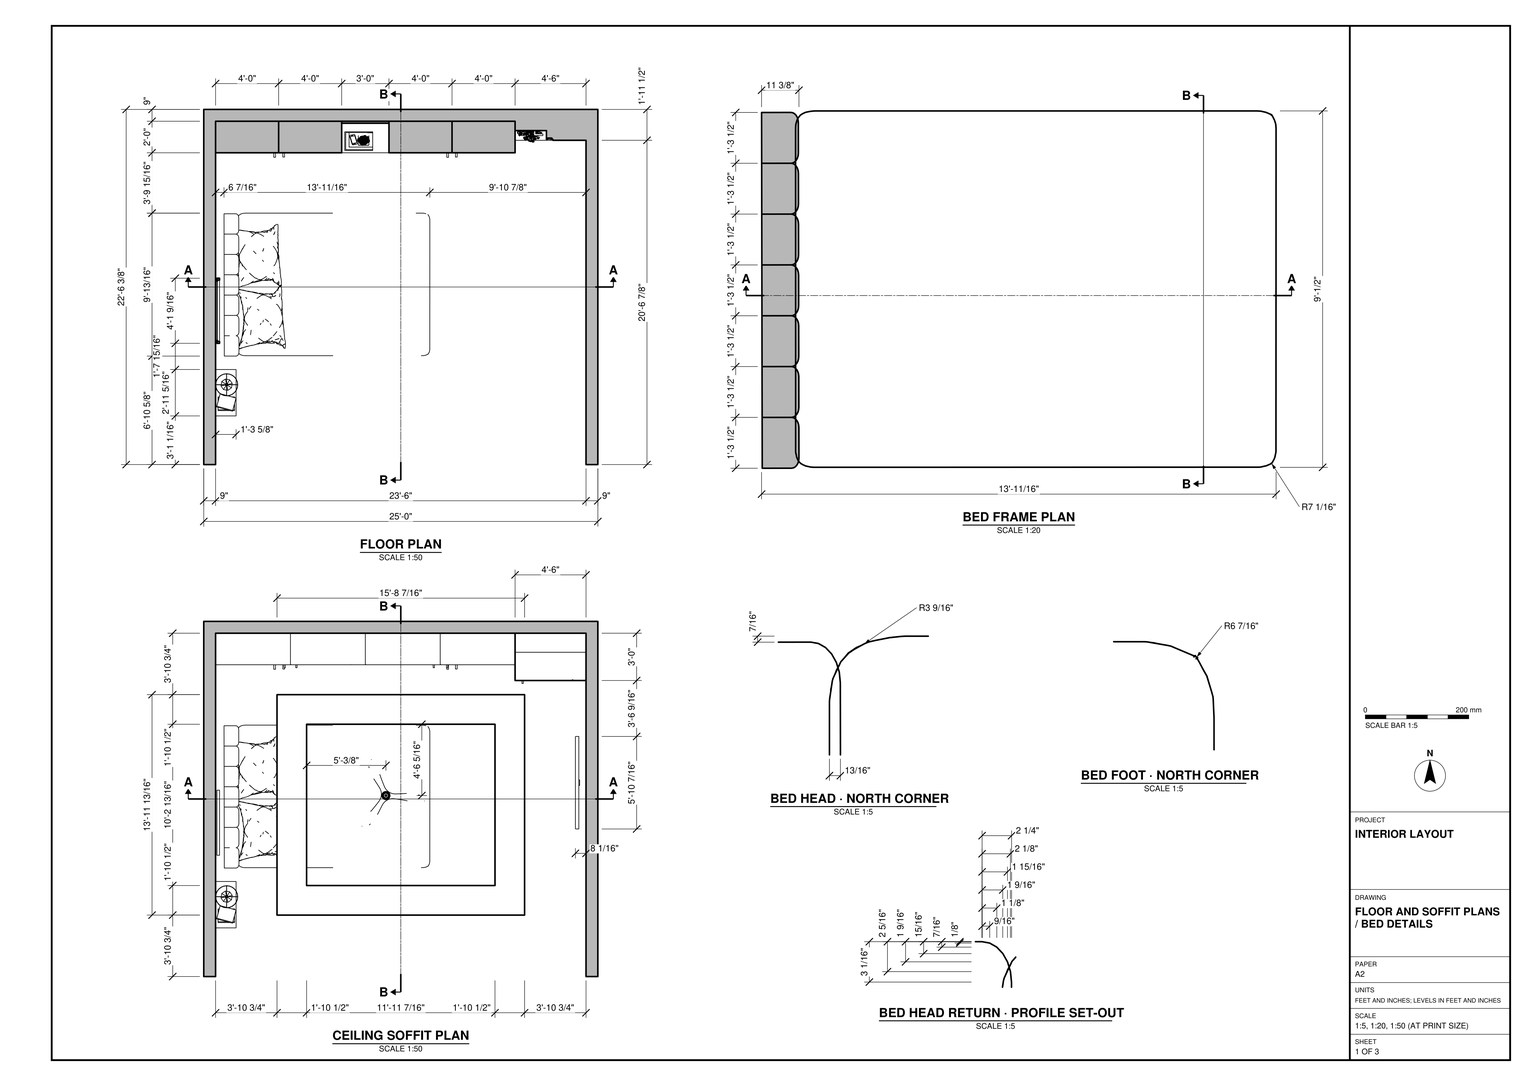
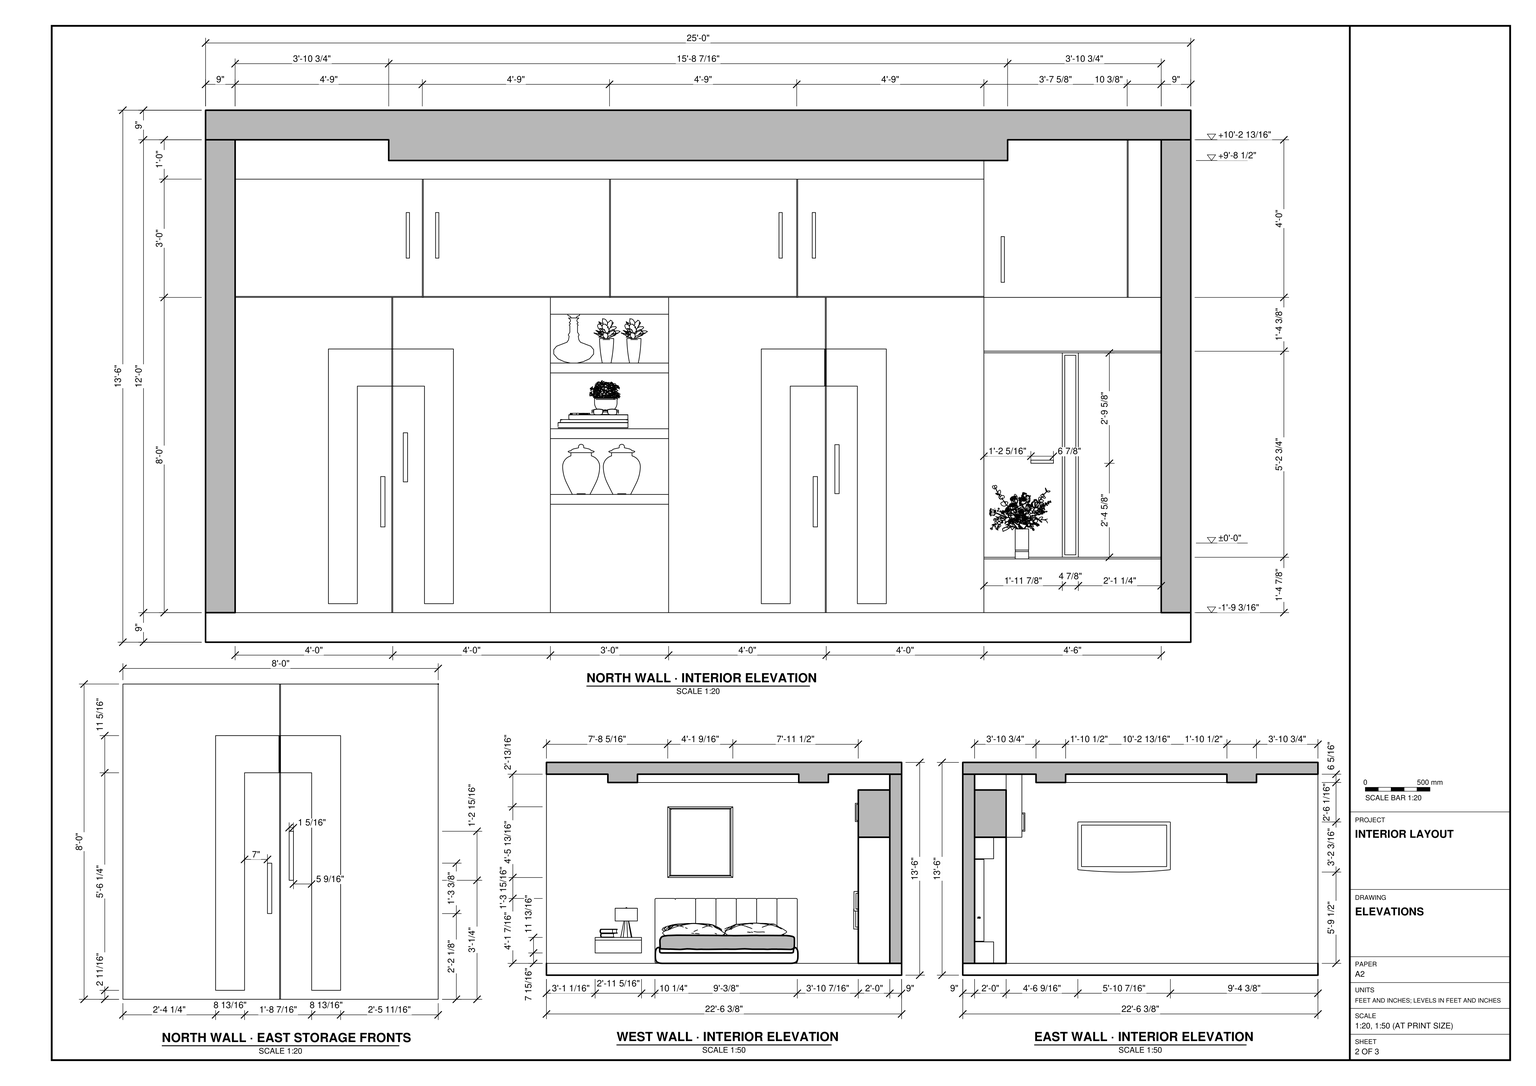
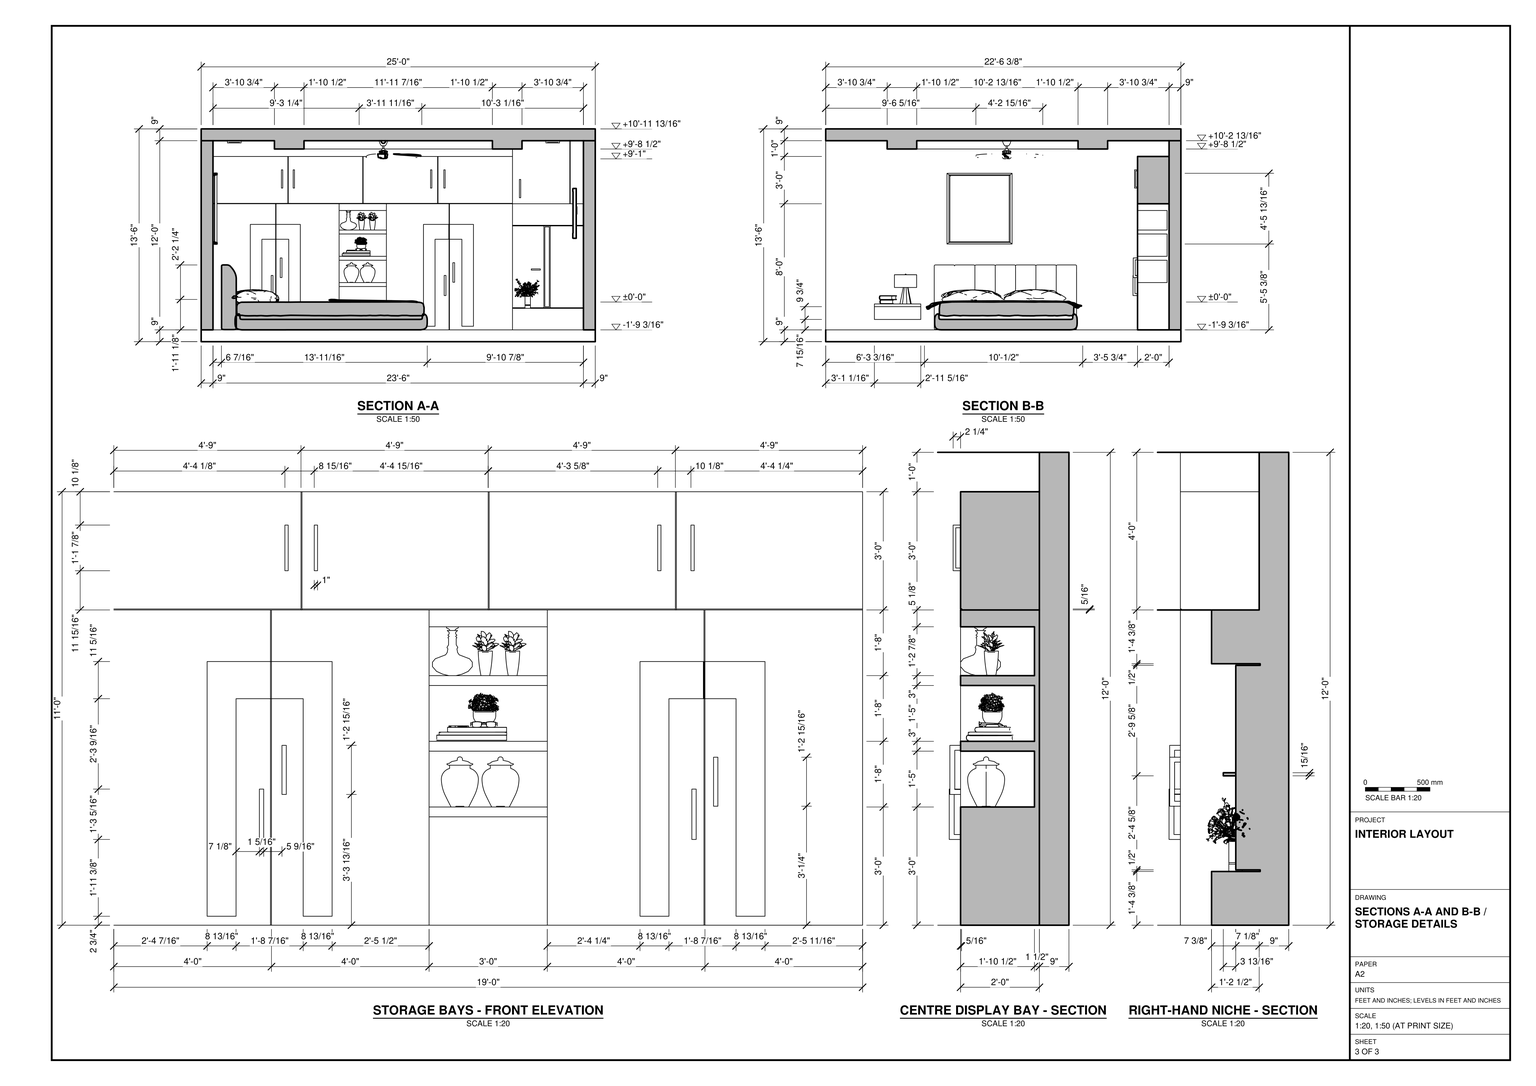
Build the bedroom interior in SketchUp from task_files/diagram_01.pdf. Work in feet and inches. The model is 25'-0" wide from west to east, 22'-6 3/8" deep from north to south and 13'-6" high. Use the single storey datum of ±0'-0" shown in the sections.

Form the floor slab, ceiling slab and 9" walls on the north, east and west sides, leaving the south side open as drawn. Follow the ceiling soffit plan and both sections to form the rectangular dropped band around the recessed centre. Place the ceiling fan within that recess at the position shown.

Run the fitted storage across the north wall. Distinguish the tall paired fronts, central display shelves, upper cupboards and stepped niche at the east end. Use the storage elevations for the front divisions, inset outlines and offset handles, and the bay sections for shelf depths and projections. Set the platform bed with its segmented head toward the west wall and its rounded foot toward the east. Include the mattress, the bedside unit south of the head, the framed panel above the bed and the screen opposite it. Decor and loose items such as lamps, cushions, plants and books may be any suitable library components, for example from 3D Warehouse.

Keep the walls, slabs and soffit, and each furniture or joinery piece, in separate groups or components. Use components for repeated parts. Save one SketchUp model as output_files/bedroom_with_fitted_storage_and_a_platform_bed.skp.

# SketchUp Ruby script. Lengths in inches.
U = 1.inch
M = Sketchup.active_model
def pt(a) = Geom::Point3d.new(a.map { |v| v * U })
def face(e, loops, mat)
  f = e.add_face(loops[0].map { |a| pt(a) })
  loops[1..].each { |l| e.add_face(l.map { |a| pt(a) }).erase! }
  f.material = f.back_material = mat if mat
  f
end
# faces: each face lists its corners as indices into pts; further lists are holes
def faces(e, pts, list, mat = nil) = list.each { |f| face(e, (f[0].is_a?(Array) ? f : [f]).map { |l| l.map { |i| pts[i] } }, mat) }
# xy, xz, yz: faces in a plane at the given z, y or x. An outline is a flat list of corners, or four numbers for a rectangle; further outlines are holes
def ring(l) = l.size == 4 ? [[l[0], l[1]], [l[2], l[1]], [l[2], l[3]], [l[0], l[3]]] : l.each_slice(2).to_a
def flat(e, list, mat, &to3) = list.each { |f| face(e, (f[0].is_a?(Array) ? f : [f]).map { |l| ring(l).map { |u, v| to3.(u, v) } }, mat) }
def xy(e, z, list, mat = nil) = flat(e, list, mat) { |x, y| [x, y, z] }
def xz(e, y, list, mat = nil) = flat(e, list, mat) { |x, z| [x, y, z] }
def yz(e, x, list, mat = nil) = flat(e, list, mat) { |y, z| [x, y, z] }
def lines(e, pts, list) = list.each { |a, b| e.add_line(pt(pts[a]), pt(pts[b])) }
# prism: a flat outline (further loops are holes) pulled along v
def prism(e, loops, v, mat = nil)
  f = face(e, loops, mat); d = Geom::Vector3d.new(v.map { |x| x * U })
  f.pushpull(f.normal.samedirection?(d) ? d.length : -d.length)
end
def box(e, o, s, mat = nil) = prism(e, [[o, [o[0] + s[0], o[1], o[2]], [o[0] + s[0], o[1] + s[1], o[2]], [o[0], o[1] + s[1], o[2]]]], [0, 0, s[2]], mat)
def at(x, y, z, deg = 0) = Geom::Transformation.translation(pt([x, y, z])) * Geom::Transformation.rotation(ORIGIN, Z_AXIS, deg.degrees)
def axes(o, x, y, z) = Geom::Transformation.new([*x, 0, *y, 0, *z, 0, *pt(o).to_a, 1])
def part(name) = M.definitions.add(name)
# library, detail: a bought-in or finely detailed component or shape, given as its bounding box
def library(name, o, s) = part(name).tap { |d| box(d.entities, o, s) }
def detail(e, o, s) = box(e.add_group.entities, o, s)
def put(e, d, t, mat = nil) = e.add_instance(d, t).tap { |i| i.material = mat if mat }
def group(e, t, mat = nil) = e.add_group.tap { |g| g.transformation = t; g.material = mat if mat }.entities
root = M.entities
M.materials.add("Ceramic White").color = [255, 255, 255]
M.materials.add("Generic\#1").color = [232, 226, 159]
M.materials.add("[Color M07]").color = [58, 58, 58]
M.materials.add("[Tile Limestone Large]").color = [236, 249, 228]
M.materials.add("[Wood Bamboo]").color = [153, 90, 37]
c1 = library("Flower+Arrangement",[-12.45,-7.69,-0.03],[24.36,19.47,24.52])
c2 = library("00000871-book1",[-1.17,-10.85,-0.02],[14.86,13.34,6.32])
c3 = library("Lidded jar",[0,0,0],[13.42,13.42,18.18])
c4 = library("books",[6.19,-1.3125,-0.22],[15.35,11.9,12.07])
c5 = library("Lamp+10 (1)",[0,0,0],[16.92,16.92,22.79])
c6 = library("Untitled",[82.71,28.87,-11.8125],[39.77,1.97,25.2])
c7 = library("sri rejeki",[-5.27,-3.99,-0.125],[72.84,72.27,70.8])
c8 = library("Tlon Light 450 Ceiling 152 006",[-8.86,-8.86,-3.78],[17.72,17.72,3.56])
c9 = library("Avation+Styled+Ceiling+Fan_JSB",[-19.77,-29.63,-13.8125],[51.59,58.16,13.8125])
c10 = library("Group\#9",[0,0,0],[159.9,159.9,209.38])
c11 = library("Group\#50",[-3.59,0,-0.01],[91.02,69.39,39.65])
c12 = library("Group\#4",[0,0,0],[11.81,11.74,23.62])
c13 = library("Group\#16",[-1.58,-1.2,0],[21.85,21.68,32.68])
c14 = part("Agrupar\#12")
xy(c14.entities,0,[[0,13.9375,0,31.5,0.51,30.98,0.51,14.45]])
xy(c14.entities,1.0625,[[0.51,14.45,0.51,30.98,0.79,30.71,0.79,14.72]])
xy(c14.entities,1.26,[[0,13.9375,0.79,14.72,0.79,30.71,0,31.5]])
yz(c14.entities,0,[[13.9375,0,31.5,1.26]])
yz(c14.entities,0.51,[[14.45,0,30.98,1.0625]])
yz(c14.entities,0.79,[[14.72,1.0625,30.71,1.26]])
p = [[0.79,14.72,1.26],[0,13.9375,1.26],[0,13.9375,0],[0.51,14.45,0],[0.51,14.45,1.0625],[0.79,14.72,1.0625],
  [0,31.5,1.26],[0.79,30.71,1.26],[0.79,30.71,1.0625],[0.51,30.98,1.0625],[0.51,30.98,0],[0,31.5,0]]
faces(c14.entities,p,[[0,1,2,3,4,5],[6,7,8,9,10,11]])
c15 = part("Agrupar\#31")
xy(c15.entities,0,[[0,6.85,0,31.5,0.51,30.98,0.51,7.36]])
xy(c15.entities,1.0625,[[0.51,7.36,0.51,30.98,0.79,30.71,0.79,7.64]])
xy(c15.entities,1.26,[[0,6.85,0.79,7.64,0.79,30.71,0,31.5]])
yz(c15.entities,0,[[6.85,0,31.5,1.26]])
yz(c15.entities,0.51,[[7.36,0,30.98,1.0625]])
yz(c15.entities,0.79,[[7.64,1.0625,30.71,1.26]])
p = [[0.79,7.64,1.26],[0,6.85,1.26],[0,6.85,0],[0.51,7.36,0],[0.51,7.36,1.0625],[0.79,7.64,1.0625],
  [0,31.5,1.26],[0.79,30.71,1.26],[0.79,30.71,1.0625],[0.51,30.98,1.0625],[0.51,30.98,0],[0,31.5,0]]
faces(c15.entities,p,[[0,1,2,3,4,5],[6,7,8,9,10,11]])
c16 = part("Agrupar\#29")
put(c16.entities,c14,at(0,-13.9375,0))
put(c16.entities,c15,at(31.5,0,0,90))
put(c16.entities,c14,at(24.65,31.5,0,-180))
put(c16.entities,c15,at(-6.85,17.56,0,-90))
xy(root,-9,[[0,0,300,270.375]],"[Tile Limestone Large]")
xy(root,0,[[0,0,9,0,9,261.375,237,261.375,237,246.875,291,246.875,291,0,300,0,300,270.375,0,270.375],[9,237.375,56.7,237.375,56.7,237.68,57,237.68,57,261.375,9,261.375],[57,237.375,105,261.375],[105,237.375,141,261.375],[141,237.375,188.7,237.375,188.7,237.68,189,237.68,189,261.375,141,261.375],
  [189,237.375,237,261.375]])
xy(root,7.92,[[9,37.05,24.62,72.37]])
xy(root,16.36,[[260.875,246.875,263.875,261.67],[263.875,246.875,291,261.67]])
xy(root,16.36,[[237,246.875,260.875,261.67]],"[Wood Bamboo]")
xy(root,16.86,[[265.75,246.875,265.75,251.4375,263.875,261.67,291,261.67,291,246.875],[260.875,247.625,260.875,261.67,263.875,261.67,265.75,251.4375,265.75,247.625],[237,254.25,260.875,261.67]])
xy(root,17.61,[[261.625,247.625,265,248.5625]])
xy(root,17.67,[[9,37.05,24.62,72.37]])
xy(root,19.73,[[9,37.05,24.62,72.37]])
xy(root,26.11,[[53.32,233.93,54.64,237.375],[185.01,233.93,186.32,237.375]],"[Color M07]")
xy(root,27.61,[[53.32,235.43,54.64,237.375],[185.01,235.43,186.32,237.375]],"[Color M07]")
xy(root,36,[[105,237.375,141,259.875]],"[Wood Bamboo]")
xy(root,36.23,[[191.62,234.13,192.93,237.375]],"[Color M07]")
xy(root,37.73,[[191.62,235.63,192.93,237.375]],"[Color M07]")
xy(root,39.82,[[60.21,234.12,61.52,237.375]],"[Color M07]")
xy(root,39.95,[[53.32,235.43,54.64,237.375],[185.01,235.43,186.32,237.375]],"[Color M07]")
xy(root,41.32,[[60.21,235.62,61.52,237.375]],"[Color M07]")
xy(root,41.45,[[53.32,233.93,54.64,237.375],[185.01,233.93,186.32,237.375]],"[Color M07]")
xy(root,45.49,[[251.3125,250.45,251.3125,254.25,252.625,254.25,252.625,251.76,258.18,251.76,258.18,250.45]],"[Color M07]")
xy(root,46.44,[[251.3125,250.45,258.18,250.45,258.18,251.76,252.625,251.76,252.625,254.25,251.3125,254.25]],"[Color M07]")
xy(root,49.66,[[191.62,235.63,192.93,237.375]],"[Color M07]")
xy(root,51.16,[[191.62,234.13,192.93,237.375]],"[Color M07]")
xy(root,53,[[105,237.375,141,259.875]])
xy(root,53.27,[[60.21,235.62,61.52,237.375]])
xy(root,54.77,[[60.21,234.12,61.52,237.375]],"[Color M07]")
xy(root,56,[[105,237.375,141,259.875]],"[Wood Bamboo]")
xy(root,73,[[105,237.375,141,259.875]])
xy(root,76,[[105,237.375,141,259.875]],"[Wood Bamboo]")
xy(root,78.375,[[261.625,247.625,265,248.5625]])
xy(root,79.125,[[265.75,246.875,291,246.875,291,261.67,263.875,261.67,265.75,251.4375],[260.875,247.625,265.75,247.625,265.75,251.4375,263.875,261.67,260.875,261.67],[237,254.25,260.875,261.67]])
xy(root,79.625,[[237,246.875,260.875,261.67],[260.875,246.875,263.875,261.67],[263.875,246.875,291,261.67]],"[Wood Bamboo]")
xy(root,90.875,[[105,237.375,141,259.875]])
xy(root,96,[[9,237.375,56.7,237.68],[57,237.375,66,237.68],[66,237.375,66.3,237.68],[66.3,237.375,105,237.68],[105,237.375,123,237.68],
  [123,237.375,123.3,237.68],[123.3,237.375,141,237.68],[141,237.375,180,237.68],[180,237.375,180.3,237.68],[180.3,237.375,188.7,237.68],
  [189,237.375,237,237.68],[9,237.68,57,261.375],[57,237.68,66,261.375],[66,237.68,105,261.375],[105,237.68,123,261.375],
  [123,237.68,141,261.375],[141,237.68,180,261.375],[180,237.68,189,261.375],[189,237.68,237,261.375],[237,246.875,291,261.375]])
xy(root,96,[[237,225.375,237,246.875,291,246.875,291,225.375,280.9375,225.375,280.9375,225.68,280.64,225.68,280.64,225.375]],"[Wood Bamboo]")
xy(root,96.3,[[9,237.375,57,237.68],[57,237.375,66,237.68],[66.3,237.375,105,237.68],[105,237.375,123,237.68],[123.3,237.375,141,237.68],
  [141,237.375,180,237.68],[180.3,237.375,189,237.68],[189,237.375,237,237.68]])
xy(root,100.58,[[242.25,223.09,243.25,225.375]],"[Color M07]")
xy(root,101.4,[[242.25,223.9,243.25,225.375]],"[Color M07]")
xy(root,107.95,[[61.1,235.11,62.1,237.375],[70.03,235.11,71.03,237.375],[174.61,235.11,175.61,237.375],[184.73,235.11,185.73,237.375]],"[Color M07]")
xy(root,108.76,[[61.1,235.92,62.1,237.375],[70.03,235.92,71.03,237.375],[174.61,235.92,175.61,237.375],[184.73,235.92,185.73,237.375]],"[Color M07]")
xy(root,113.71,[[242.25,223.9,243.25,225.375]])
xy(root,114.52,[[242.25,223.09,243.25,225.375]],"[Color M07]")
xy(root,121.04,[[61.1,235.92,62.1,237.375],[70.03,235.92,71.03,237.375]])
xy(root,121.04,[[174.61,235.92,175.61,237.375],[184.73,235.92,185.73,237.375]],"[Color M07]")
xy(root,121.85,[[184.73,235.11,185.73,237.375]])
xy(root,121.85,[[61.1,235.11,62.1,237.375],[70.03,235.11,71.03,237.375],[174.61,235.11,175.61,237.375]],"[Color M07]")
xy(root,132,[[9,237.375,66,261.375],[66.3,237.375,123,237.375,123,261.375,66,261.375,66,237.68,66.3,237.68],[123.3,237.375,180,237.375,180,261.375,123,261.375,123,237.68,123.3,237.68],[180.3,237.375,237,237.375,237,261.375,180,261.375,180,237.68,180.3,237.68]],"[Wood Bamboo]")
xy(root,137.6875,[[[55.77,46.77,244.23,214.61],[78.29,69.29,221.71,192.08]]],"Generic\#1")
xy(root,144,[[0,0,0,270.375,300,270.375,300,0,291,0,291,261.375,9,261.375,9,0],[237,225.375,237,261.375,291,261.375,291,225.375,280.9375,225.375,280.9375,225.68,280.64,225.68,280.64,225.375]])
xy(root,144,[[[9,0,9,261.375,237,261.375,237,225.375,280.64,225.375,280.64,225.68,280.9375,225.68,280.9375,225.375,291,225.375,291,0],[55.77,46.77,244.23,214.61]],[78.29,69.29,221.71,192.08]],"Generic\#1")
xy(root,153,[[0,0,300,270.375]])
xz(root,0,[[0,-9,300,0],[0,0,9,144],[291,0,300,144],[0,144,300,153]])
xz(root,37.05,[[9,7.92,24.62,17.67],[9,17.67,24.62,19.73]])
xz(root,46.77,[[55.77,137.6875,244.23,144]],"Generic\#1")
xz(root,69.29,[[78.29,137.6875,221.71,144]])
xz(root,72.37,[[9,7.92,24.62,17.67],[9,17.67,24.62,19.73]])
xz(root,192.08,[[78.29,137.6875,221.71,144]],"Generic\#1")
xz(root,214.61,[[55.77,137.6875,190.23,144],[190.23,137.6875,234.17,144],[234.17,137.6875,244.23,144]])
xz(root,223.09,[[242.25,100.58,243.25,114.52]],"[Color M07]")
xz(root,223.9,[[242.25,101.4,243.25,113.71]])
xz(root,225.375,[[242.25,113.71,243.25,114.52]])
xz(root,225.375,[[[237,96,280.64,144],[242.25,113.71,243.25,114.52],[242.25,100.58,243.25,101.4]],[280.9375,96,291,144]],"[Wood Bamboo]")
xz(root,225.68,[[280.64,96,280.9375,144]])
xz(root,233.93,[[53.32,26.11,54.64,41.45],[185.01,26.11,186.32,41.45]],"[Color M07]")
xz(root,234.12,[[60.21,39.82,61.52,54.77]],"[Color M07]")
xz(root,234.13,[[191.62,36.23,192.93,51.16]],"[Color M07]")
xz(root,235.11,[[61.1,107.95,62.1,121.85],[70.03,107.95,71.03,121.85],[174.61,107.95,175.61,121.85],[184.73,107.95,185.73,121.85]],"[Color M07]")
xz(root,235.43,[[53.32,27.61,54.64,39.95],[185.01,27.61,186.32,39.95]])
xz(root,235.62,[[60.21,41.32,61.52,53.27]])
xz(root,235.63,[[191.62,37.73,192.93,49.66]])
xz(root,235.92,[[61.1,108.76,62.1,121.04],[70.03,108.76,71.03,121.04],[174.61,108.76,175.61,121.04],[184.73,108.76,185.73,121.04]])
xz(root,237.375,[[37.41,2.73,46.22,2.73,46.22,68.98,56.7,68.98,56.7,80.29,37.41,80.29],[66.66,2.73,75.47,2.73,75.47,80.29,57,80.29,57,68.98,66.66,68.98],[169.22,2.73,178.04,2.73,178.04,68.98,188.51,68.98,188.51,80.29,169.22,80.29],[198.47,2.73,207.29,2.73,207.29,80.29,189,80.29,189,68.98,198.47,68.98],[53.32,39.95,54.64,41.45],
  [185.01,39.95,186.32,41.45],[191.62,49.66,192.93,51.16],[60.21,53.27,61.52,54.77],[56.7,68.98,57,80.29],[188.8125,68.98,189,80.29],
  [61.1,121.04,62.1,121.85],[70.03,121.04,71.03,121.85],[174.61,121.04,175.61,121.85],[184.73,121.04,185.73,121.85]])
xz(root,237.375,[[[9,0,56.7,0,56.7,68.98,46.22,68.98,46.22,2.73,37.41,2.73,37.41,80.29,56.7,80.29,56.7,96,9,96],[53.32,39.95,54.64,41.45],[53.32,26.11,54.64,27.61]],[[57,0,105,0,105,96,57,96,57,80.29,75.47,80.29,75.47,2.73,66.66,2.73,66.66,68.98,57,68.98],[60.21,53.27,61.52,54.77],[60.21,39.82,61.52,41.32]],[105,0,141,33],[[141,0,188.7,96],[169.22,2.73,169.22,80.29,188.51,80.29,188.51,68.98,178.04,68.98,178.04,2.73],[185.01,39.95,186.32,41.45],[185.01,26.11,186.32,27.61]],[[189,0,237,0,237,96,189,96,189,80.29,207.29,80.29,207.29,2.73,198.47,2.73,198.47,68.98,189,68.98],[191.62,49.66,192.93,51.16],[191.62,36.23,192.93,37.73]],
  [105,33,141,36],[105,53,141,56],[105,73,141,76],[105,90.875,141,96],[[9,96.3,66,132],[61.1,121.04,62.1,121.85],[61.1,107.95,62.1,108.76]],
  [[66.3,96.3,123,132],[70.03,121.04,71.03,121.85],[70.03,107.95,71.03,108.76]],[[123.3,96.3,180,132],[174.61,121.04,175.61,121.85],[174.61,107.95,175.61,108.76]],[[180.3,96.3,237,132],[184.73,121.04,185.73,121.85],[184.73,107.95,185.73,108.76]]],"[Wood Bamboo]")
xz(root,237.68,[[56.7,0,57,96],[188.7,0,189,96],[9,96,66,96.3],[66,96,66.3,132],[66.3,96,123,96.3],
  [123,96,123.3,132],[123.3,96,180,96.3],[180,96,180.3,132],[180.3,96,237,96.3]])
xz(root,246.875,[[237,0,291,16.36],[265.75,16.86,291,79.125],[237,79.625,291,96]],"[Wood Bamboo]")
xz(root,247.625,[[[260.875,16.86,265.75,79.125],[261.625,17.61,265,78.375]]],"[Wood Bamboo]")
xz(root,248.5625,[[261.625,17.61,265,78.375]],"[Wood Bamboo]")
xz(root,250.45,[[251.3125,45.49,258.18,46.44]],"[Color M07]")
xz(root,251.76,[[252.625,45.49,258.18,46.44]])
xz(root,254.25,[[251.3125,45.49,252.625,46.44]])
xz(root,254.25,[[[237,16.86,260.875,79.125],[251.3125,45.49,252.625,46.44]]],"[Wood Bamboo]")
xz(root,259.875,[[105,36,141,53],[105,56,141,73],[105,76,141,90.875]],"[Wood Bamboo]")
xz(root,261.375,[[9,0,57,96],[57,0,105,96],[105,0,141,96],[141,0,189,96],[189,0,237,96],
  [9,96,66,132],[66,96,123,132],[123,96,180,132],[180,96,237,132],[237,96,291,144]])
xz(root,261.375,[[9,132,237,144]],"[Wood Bamboo]")
xz(root,261.67,[[237,16.36,291,16.86],[237,79.125,291,79.625]])
xz(root,270.375,[[0,0,300,144],[0,144,300,153]])
xz(root,270.375,[[0,-9,300,0]],"Generic\#1")
yz(root,0,[[0,-9,270.375,0],[0,0,270.375,144],[0,144,270.375,153]])
yz(root,9,[[237.375,0,261.375,96],[37.05,7.92,72.37,17.67],[37.05,17.67,72.37,19.73],[237.68,96,261.375,96,261.375,132,237.375,132,237.375,96.3,237.68,96.3]])
yz(root,9,[[[0,0,237.375,0,237.375,96,237.68,96,237.68,96.3,237.375,96.3,237.375,132,261.375,132,261.375,144,0,144],[37.05,7.92,72.37,19.73]]],"Generic\#1")
yz(root,24.62,[[37.05,7.92,72.37,17.67],[37.05,17.67,72.37,19.73]])
yz(root,53.32,[[233.93,26.11,233.93,41.45,237.375,41.45,237.375,39.95,235.43,39.95,235.43,27.61,237.375,27.61,237.375,26.11]],"[Color M07]")
yz(root,54.64,[[233.93,26.11,237.375,26.11,237.375,27.61,235.43,27.61,235.43,39.95,237.375,39.95,237.375,41.45,233.93,41.45]],"[Color M07]")
yz(root,55.77,[[46.77,137.6875,214.61,144]])
yz(root,56.7,[[237.375,0,237.68,96]])
yz(root,57,[[237.375,0,237.68,96],[237.68,0,261.375,96]])
yz(root,60.21,[[234.12,39.82,234.12,54.77,237.375,54.77,237.375,53.27,235.62,53.27,235.62,41.32,237.375,41.32,237.375,39.82]],"[Color M07]")
yz(root,61.1,[[235.11,107.95,235.11,121.85,237.375,121.85,237.375,121.04,235.92,121.04,235.92,108.76,237.375,108.76,237.375,107.95]],"[Color M07]")
yz(root,61.52,[[234.12,39.82,237.375,39.82,237.375,41.32,235.62,41.32,235.62,53.27,237.375,53.27,237.375,54.77,234.12,54.77]],"[Color M07]")
yz(root,62.1,[[235.11,107.95,237.375,107.95,237.375,108.76,235.92,108.76,235.92,121.04,237.375,121.04,237.375,121.85,235.11,121.85]],"[Color M07]")
yz(root,66,[[237.68,96,261.375,132],[237.375,96.3,237.68,132]])
yz(root,66.3,[[237.375,96.3,237.68,132]])
yz(root,70.03,[[235.11,107.95,235.11,121.85,237.375,121.85,237.375,121.04,235.92,121.04,235.92,108.76,237.375,108.76,237.375,107.95]],"[Color M07]")
yz(root,71.03,[[235.11,107.95,237.375,107.95,237.375,108.76,235.92,108.76,235.92,121.04,237.375,121.04,237.375,121.85,235.11,121.85]],"[Color M07]")
yz(root,78.29,[[69.29,137.6875,192.08,144]],"Generic\#1")
yz(root,105,[[237.375,0,261.375,0,261.375,96,237.375,96,237.375,90.875,259.875,90.875,259.875,76,237.375,76,237.375,73,259.875,73,259.875,56,237.375,56,237.375,53,259.875,53,259.875,36,237.375,36]])
yz(root,105,[[237.375,36,259.875,53],[237.375,56,259.875,73],[237.375,76,259.875,90.875]],"[Wood Bamboo]")
yz(root,123,[[237.68,96,261.375,132],[237.375,96.3,237.68,132]])
yz(root,123.3,[[237.375,96.3,237.68,132]])
yz(root,141,[[237.375,0,261.375,0,261.375,96,237.375,96,237.375,90.875,259.875,90.875,259.875,76,237.375,76,237.375,73,259.875,73,259.875,56,237.375,56,237.375,53,259.875,53,259.875,36,237.375,36]])
yz(root,141,[[237.375,36,259.875,53],[237.375,56,259.875,73],[237.375,76,259.875,90.875]],"[Wood Bamboo]")
yz(root,174.61,[[235.11,107.95,235.11,121.85,237.375,121.85,237.375,121.04,235.92,121.04,235.92,108.76,237.375,108.76,237.375,107.95]],"[Color M07]")
yz(root,175.61,[[235.11,107.95,237.375,107.95,237.375,108.76,235.92,108.76,235.92,121.04,237.375,121.04,237.375,121.85,235.11,121.85]],"[Color M07]")
yz(root,180,[[237.68,96,261.375,132],[237.375,96.3,237.68,132]])
yz(root,180.3,[[237.375,96.3,237.68,132]])
yz(root,184.73,[[235.11,107.95,235.11,121.85,237.375,121.85,237.375,121.04,235.92,121.04,235.92,108.76,237.375,108.76,237.375,107.95]],"[Color M07]")
yz(root,185.01,[[233.93,26.11,233.93,41.45,237.375,41.45,237.375,39.95,235.43,39.95,235.43,27.61,237.375,27.61,237.375,26.11]],"[Color M07]")
yz(root,185.73,[[235.11,107.95,237.375,107.95,237.375,108.76,235.92,108.76,235.92,121.04,237.375,121.04,237.375,121.85,235.11,121.85]],"[Color M07]")
yz(root,186.32,[[233.93,26.11,237.375,26.11,237.375,27.61,235.43,27.61,235.43,39.95,237.375,39.95,237.375,41.45,233.93,41.45]],"[Color M07]")
yz(root,188.7,[[237.375,0,237.68,96]])
yz(root,189,[[237.375,0,237.68,96],[237.68,0,261.375,96]])
yz(root,191.62,[[234.13,36.23,234.13,51.16,237.375,51.16,237.375,49.66,235.63,49.66,235.63,37.73,237.375,37.73,237.375,36.23]],"[Color M07]")
yz(root,192.93,[[234.13,36.23,237.375,36.23,237.375,37.73,235.63,37.73,235.63,49.66,237.375,49.66,237.375,51.16,234.13,51.16]],"[Color M07]")
yz(root,221.71,[[69.29,137.6875,192.08,144]],"Generic\#1")
yz(root,237,[[246.875,0,261.375,16.36],[261.375,16.36,261.67,16.86],[254.25,16.86,261.375,79.125],[261.375,79.125,261.67,79.625],[246.875,79.625,261.375,96],
  [237.68,96,237.68,96.3,237.375,96.3,237.375,132,261.375,132,261.375,96]])
yz(root,237,[[237.375,0,246.875,0,246.875,16.36,261.375,16.36,261.375,16.86,254.25,16.86,254.25,79.125,261.375,79.125,261.375,79.625,246.875,79.625,246.875,96,237.375,96],[225.375,96,225.375,144,237.375,144,237.375,96.3,237.68,96.3,237.68,96],[237.375,132,261.375,144]],"[Wood Bamboo]")
yz(root,242.25,[[223.09,100.58,223.09,114.52,225.375,114.52,225.375,113.71,223.9,113.71,223.9,101.4,225.375,101.4,225.375,100.58]],"[Color M07]")
yz(root,243.25,[[223.09,100.58,225.375,100.58,225.375,101.4,223.9,101.4,223.9,113.71,225.375,113.71,225.375,114.52,223.09,114.52]],"[Color M07]")
yz(root,244.23,[[46.77,137.6875,214.61,144]])
yz(root,251.3125,[[250.45,45.49,254.25,46.44]],"[Color M07]")
yz(root,252.625,[[251.76,45.49,254.25,46.44]],"[Color M07]")
yz(root,258.18,[[250.45,45.49,251.76,46.44]])
yz(root,260.875,[[247.625,16.86,254.25,79.125]],"[Wood Bamboo]")
yz(root,261.625,[[247.625,17.61,248.5625,78.375]])
yz(root,265,[[247.625,17.61,248.5625,78.375]])
yz(root,265.75,[[246.875,16.86,247.625,79.125]])
yz(root,280.64,[[225.375,96,225.68,144]])
yz(root,280.9375,[[225.375,96,225.68,144]])
yz(root,291,[[225.375,96,261.375,144]])
yz(root,291,[[0,0,0,144,225.375,144,225.375,96,246.875,96,246.875,79.625,261.67,79.625,261.67,79.125,246.875,79.125,246.875,16.86,261.67,16.86,261.67,16.36,246.875,16.36,246.875,0]],"Generic\#1")
yz(root,300,[[0,-9,270.375,0],[0,0,270.375,144],[0,144,270.375,153]])
p = [[61.58,237.375,121.39],[61.58,235.5625,121.39],[61.58,235.5625,108.41],[61.58,237.375,108.41],[70.51,235.5625,108.41],[70.51,237.375,108.41],
  [70.51,235.5625,121.39],[70.51,237.375,121.39],[175.2,235.5625,108.41],[175.2,237.375,108.41],[175.2,235.5625,121.39],[175.2,237.375,121.39],
  [185.39,235.5625,121.39],[185.39,235.5625,108.41],[185.39,237.375,108.41],[185.39,237.375,121.39],[242.8125,223.5625,114.05],[242.8125,223.5625,101.06],
  [242.8125,225.375,101.06],[242.8125,225.375,114.05],[60.58,237.375,54.08],[60.58,234.8125,54.08],[60.58,234.8125,40.52],[60.58,237.375,40.52],
  [54.01,234.8125,27],[54.01,237.375,27],[54.01,237.375,40.56],[54.01,234.8125,40.56],[185.64,234.8125,27],[185.64,237.375,27],
  [185.64,234.8125,40.56],[185.64,237.375,40.56],[192.28,234.8125,36.92],[192.28,237.375,36.92],[192.28,234.8125,50.48],[192.28,237.375,50.48],
  [252.11,254.25,45.98],[252.11,251.25,45.98],[258.18,251.25,45.98],[-308.98,134.76,0],[-308.98,134.76,17.72]]
lines(root,p,[[0,1],[1,2],[2,3],[4,5],[6,4],[7,6],[8,9],[10,8],[11,10],[12,13],[13,14],[15,12],
  [16,17],[17,18],[19,16],[20,21],[21,22],[22,23],[24,25],[26,27],[27,24],[28,29],[30,28],[31,30],
  [32,33],[34,32],[35,34],[36,37],[37,38],[39,40]])
put(root,c1,at(247.14,252.9375,15.05))
put(root,c2,at(10.92,51.49,19.76))
put(root,c3,axes([108.73,239.52,36],[0.84,0,0],[0,0.84,0],[0,0,0.84]))
put(root,c4,axes([98.72,240.6875,56.53],[1.38852,0,0],[0,1.197,0],[0,0,1.197]),"[Wood Bamboo]")
put(root,c5,at(9,52.29,19.73))
put(root,c6,axes([235.58,329.28,87.38],[0,-1.7712,0],[1.64,0,0],[0,0,1.51438]))
put(root,c3,axes([121.1,239.52,36],[0.84,0,0],[0,0.84,0],[0,0,0.84]))
put(root,c7,axes([-298,146.97,21.22],[-0.36,0,0],[0,-0.36,0],[0,0,0.288]))
put(root,c8,axes([267.64,181.42,144.54],[0.59,0,0],[0,0.59,0],[0,0,0.59]))
put(root,c8,axes([267.64,120.48,144.54],[0.59,0,0],[0,0.59,0],[0,0,0.59]))
put(root,c8,axes([267.64,59.54,144.54],[0.59,0,0],[0,0.59,0],[0,0,0.59]))
put(root,c8,axes([25.2,59.54,144.54],[0.59,0,0],[0,0.59,0],[0,0,0.59]))
put(root,c8,axes([25.2,181.42,144.54],[0.59,0,0],[0,0.59,0],[0,0,0.59]))
put(root,c8,axes([25.2,120.48,144.54],[0.59,0,0],[0,0.59,0],[0,0,0.59]))
put(root,c9,at(138.68,137.79,144))
put(root,c10,axes([106.03,237.375,76],[0.0759,0,0],[0,0.0759,0],[0,0,0.0759]))
put(root,c11,axes([15.43,75.16,0.01],[1.79205,0,0],[0,1.73609,0],[0,0,1.24683]),"[Wood Bamboo]")
put(root,c12,at(-314.89,128.89,0),"Ceramic White")
put(root,c13,axes([118.25,242.47,76],[0.4224,0,0],[0,0.4224,0],[0,0,0.4224]))
put(root,c13,axes([126.5625,242.47,76],[0.4224,0,0],[0,0.4224,0],[0,0,0.4224]))
g1 = group(root,at(12.02,92.31,65.36))
g2 = group(g1,at(-1.97,0,53.83))
yz(g2,0.31,[[2.22,-2.08,2.69,-1.72]])
put(g2,c16,axes([1.97,49.58,0],[0,0,-2.184],[0,-2.8236,0],[-1.56,0,0]))
